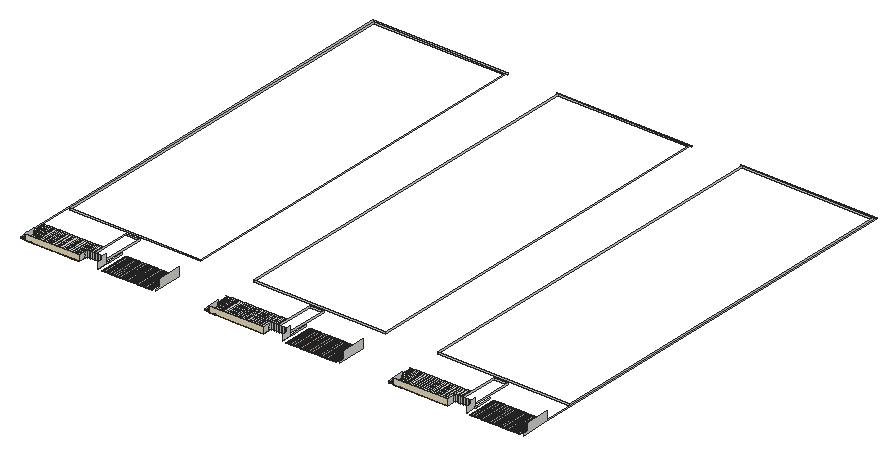
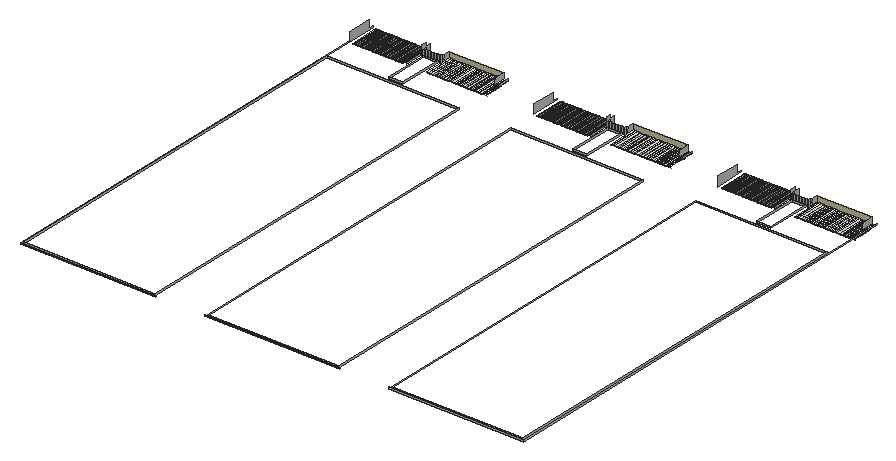
# SketchUp Ruby script. Lengths in inches.
U = 1.inch
M = Sketchup.active_model
def pt(a) = Geom::Point3d.new(a.map { |v| v * U })
def face(e, loops, mat)
  f = e.add_face(loops[0].map { |a| pt(a) })
  loops[1..].each { |l| e.add_face(l.map { |a| pt(a) }).erase! }
  f.material = f.back_material = mat if mat
  f
end
# faces: each face lists its corners as indices into pts; further lists are holes
def faces(e, pts, list, mat = nil) = list.each { |f| face(e, (f[0].is_a?(Array) ? f : [f]).map { |l| l.map { |i| pts[i] } }, mat) }
# xy, xz, yz: faces in a plane at the given z, y or x. An outline is a flat list of corners, or four numbers for a rectangle; further outlines are holes
def ring(l) = l.size == 4 ? [[l[0], l[1]], [l[2], l[1]], [l[2], l[3]], [l[0], l[3]]] : l.each_slice(2).to_a
def flat(e, list, mat, &to3) = list.each { |f| face(e, (f[0].is_a?(Array) ? f : [f]).map { |l| ring(l).map { |u, v| to3.(u, v) } }, mat) }
def xy(e, z, list, mat = nil) = flat(e, list, mat) { |x, y| [x, y, z] }
def xz(e, y, list, mat = nil) = flat(e, list, mat) { |x, z| [x, y, z] }
def yz(e, x, list, mat = nil) = flat(e, list, mat) { |y, z| [x, y, z] }
def lines(e, pts, list) = list.each { |a, b| e.add_line(pt(pts[a]), pt(pts[b])) }
# prism: a flat outline (further loops are holes) pulled along v
def prism(e, loops, v, mat = nil)
  f = face(e, loops, mat); d = Geom::Vector3d.new(v.map { |x| x * U })
  f.pushpull(f.normal.samedirection?(d) ? d.length : -d.length)
end
def box(e, o, s, mat = nil) = prism(e, [[o, [o[0] + s[0], o[1], o[2]], [o[0] + s[0], o[1] + s[1], o[2]], [o[0], o[1] + s[1], o[2]]]], [0, 0, s[2]], mat)
def at(x, y, z, deg = 0) = Geom::Transformation.translation(pt([x, y, z])) * Geom::Transformation.rotation(ORIGIN, Z_AXIS, deg.degrees)
def axes(o, x, y, z) = Geom::Transformation.new([*x, 0, *y, 0, *z, 0, *pt(o).to_a, 1])
def part(name) = M.definitions.add(name)
# library, detail: a bought-in or finely detailed component or shape, given as its bounding box
def library(name, o, s) = part(name).tap { |d| box(d.entities, o, s) }
def detail(e, o, s) = box(e.add_group.entities, o, s)
def put(e, d, t, mat = nil) = e.add_instance(d, t).tap { |i| i.material = mat if mat }
def group(e, t, mat = nil) = e.add_group.tap { |g| g.transformation = t; g.material = mat if mat }.entities
root = M.entities
M.materials.add("[Color D01]").color = [237, 225, 189]
M.materials.add("[Wood Veneer 01]").color = [51, 28, 15]
xy(root,379.5625,[[409.32,246.64,413.74,361.27],[415.32,246.64,419.74,361.27],[421.32,246.64,425.74,361.27],[427.32,246.64,431.74,361.27],[433.32,246.64,437.74,361.27],
  [439.32,246.64,443.74,361.27],[445.32,246.64,449.74,361.27],[451.32,246.64,455.74,361.27],[457.32,246.64,461.74,361.27],[463.32,246.64,467.74,361.27],
  [469.32,246.64,473.74,361.27],[475.32,246.64,479.74,361.27],[481.32,246.64,485.74,361.27],[487.32,246.64,491.74,361.27],[493.32,246.64,497.74,361.27],
  [499.32,246.64,503.74,361.27],[1142.89,246.64,1147.3,361.27],[1148.89,246.64,1153.3,361.27],[1154.89,246.64,1159.3,361.27],[1160.89,246.64,1165.3,361.27],
  [1166.89,246.64,1171.3,361.27],[1172.89,246.64,1177.3,361.27],[1178.89,246.64,1183.3,361.27],[1184.89,246.64,1189.3,361.27],[1190.89,246.64,1195.3,361.27],
  [1196.89,246.64,1201.3,361.27],[1202.89,246.64,1207.3,361.27],[1208.89,246.64,1213.3,361.27],[1214.89,246.64,1219.3,361.27],[1220.89,246.64,1225.3,361.27],
  [1226.89,246.64,1231.3,361.27],[1232.89,246.64,1237.3,361.27],[1876.45,246.64,1880.86,361.27],[1882.45,246.64,1886.86,361.27],[1888.45,246.64,1892.86,361.27],
  [1894.45,246.64,1898.86,361.27],[1900.45,246.64,1904.86,361.27],[1906.45,246.64,1910.86,361.27],[1912.45,246.64,1916.86,361.27],[1918.45,246.64,1922.86,361.27],
  [1924.45,246.64,1928.86,361.27],[1930.45,246.64,1934.86,361.27],[1936.45,246.64,1940.86,361.27],[1942.45,246.64,1946.86,361.27],[1948.45,246.64,1952.86,361.27],
  [1954.45,246.64,1958.86,361.27],[1960.45,246.64,1964.86,361.27],[1966.45,246.64,1970.86,361.27]],"[Wood Veneer 01]")
xy(root,380.0625,[[505.32,246.64,509.74,361.27],[511.32,246.64,515.74,361.27],[517.32,246.64,521.74,361.27],[523.32,246.64,527.74,361.27],[529.32,246.64,533.74,361.27],
  [535.32,246.64,539.74,361.27],[541.32,246.64,545.74,361.27],[547.32,246.64,551.74,361.27],[553.32,246.64,557.74,361.27],[559.32,246.64,563.74,361.27],
  [565.32,246.64,569.74,361.27],[1238.89,246.64,1243.3,361.27],[1244.89,246.64,1249.3,361.27],[1250.89,246.64,1255.3,361.27],[1256.89,246.64,1261.3,361.27],
  [1262.89,246.64,1267.3,361.27],[1268.89,246.64,1273.3,361.27],[1274.89,246.64,1279.3,361.27],[1280.89,246.64,1285.3,361.27],[1286.89,246.64,1291.3,361.27],
  [1292.89,246.64,1297.3,361.27],[1298.89,246.64,1303.3,361.27],[1972.45,246.64,1976.86,361.27],[1978.45,246.64,1982.86,361.27],[1984.45,246.64,1988.86,361.27],
  [1990.45,246.64,1994.86,361.27],[1996.45,246.64,2000.86,361.27],[2002.45,246.64,2006.86,361.27],[2008.45,246.64,2012.86,361.27],[2014.45,246.64,2018.86,361.27],
  [2020.45,246.64,2024.86,361.27],[2026.45,246.64,2030.86,361.27],[2032.45,246.64,2036.86,361.27]],"[Wood Veneer 01]")
xy(root,380.1875,[[571.32,246.64,575.74,361.27],[577.32,246.64,581.74,361.27],[583.32,246.64,587.74,361.27],[589.32,246.64,593.74,361.27],[595.32,246.64,599.74,361.27],
  [601.32,246.64,605.74,361.27],[1304.89,246.64,1309.3,361.27],[1310.89,246.64,1315.3,361.27],[1316.89,246.64,1321.3,361.27],[1322.89,246.64,1327.3,361.27],
  [1328.89,246.64,1333.3,361.27],[1334.89,246.64,1339.3,361.27],[2038.45,246.64,2042.86,361.27],[2044.45,246.64,2048.86,361.27],[2050.45,246.64,2054.86,361.27],
  [2056.45,246.64,2060.86,361.27],[2062.45,246.64,2066.86,361.27],[2068.45,246.64,2072.86,361.27]],"[Wood Veneer 01]")
xy(root,380.6875,[[100.08,246.64,100.18,361.27],[100.18,246.64,105.12,361.27],[105.12,246.64,108.49,361.27],[108.49,246.64,113.53,361.27],[113.53,246.64,116.9,361.27],
  [116.9,246.64,121.94,361.27],[121.94,246.64,125.32,361.27],[130.35,246.64,133.73,361.27],[133.73,246.64,138.77,361.27],[138.77,246.64,142.14,361.27],
  [142.14,246.64,147.18,361.27],[147.18,246.64,150.55,361.27],[150.55,246.64,155.59,361.27],[155.59,246.64,158.97,361.27],[158.97,246.64,164.01,361.27],
  [164.01,246.64,167.38,361.27],[167.38,246.64,172.42,361.27],[172.42,246.64,175.79,361.27],[175.79,246.64,180.83,361.27],[180.83,246.64,184.21,361.27],
  [184.21,246.64,189.24,361.27],[189.24,246.64,192.62,361.27],[192.62,246.64,197.66,361.27],[197.66,246.64,201.03,361.27],[201.03,246.64,206.07,361.27],
  [206.07,246.64,209.44,361.27],[209.44,246.64,214.48,361.27],[214.48,246.64,217.86,361.27],[217.86,246.64,222.89,361.27],[222.89,246.64,226.27,361.27],
  [226.27,246.64,231.31,361.27],[231.31,246.64,234.68,361.27],[234.68,246.64,239.72,361.27],[239.72,246.64,243.1,361.27],[243.1,246.64,248.13,361.27],
  [248.13,246.64,251.51,361.27],[251.51,246.64,256.55,361.27],[256.55,246.64,259.92,361.27],[259.92,246.64,264.96,361.27],[264.96,246.64,268.33,361.27],
  [268.33,246.64,273.37,361.27],[273.37,246.64,276.75,361.27],[276.75,246.64,281.78,361.27],[281.78,246.64,285.16,361.27],[285.16,246.64,290.2,361.27],
  [290.2,246.64,293.57,361.27],[293.57,246.64,298.61,361.27],[298.61,246.64,301.98,361.27],[301.98,246.64,307.02,361.27],[307.02,246.64,310.4,361.27],
  [310.4,246.64,315.43,361.27],[315.43,246.64,318.81,286.21],[393.95,246.64,396.57,286.21],[413.74,246.64,415.32,361.27],[419.74,246.64,421.32,361.27],
  [425.74,246.64,427.32,361.27],[431.74,246.64,433.32,361.27],[437.74,246.64,439.32,361.27],[443.74,246.64,445.32,361.27],[449.74,246.64,451.32,361.27],
  [455.74,246.64,457.32,361.27],[461.74,246.64,463.32,361.27],[467.74,246.64,469.32,361.27],[473.74,246.64,475.32,361.27],[479.74,246.64,481.32,361.27],
  [485.74,246.64,487.32,361.27],[491.74,246.64,493.32,361.27],[497.74,246.64,499.32,361.27],[503.74,246.64,505.32,361.27],[509.74,246.64,511.32,361.27],
  [515.74,246.64,517.32,361.27],[521.74,246.64,523.32,361.27],[527.74,246.64,529.32,361.27],[533.74,246.64,535.32,361.27],[539.74,246.64,541.32,361.27],
  [545.74,246.64,547.32,361.27],[551.74,246.64,553.32,361.27],[557.74,246.64,559.32,361.27],[563.74,246.64,565.32,361.27],[569.74,246.64,571.32,361.27],
  [575.74,246.64,577.32,361.27],[581.74,246.64,583.32,361.27],[587.74,246.64,589.32,361.27],[593.74,246.64,595.32,361.27],[599.74,246.64,601.32,361.27],
  [605.74,246.64,609.07,361.27],[833.64,246.64,833.74,361.27],[833.74,246.64,838.68,361.27],[838.68,246.64,842.05,361.27],[842.05,246.64,847.09,361.27],
  [847.09,246.64,850.47,361.27],[850.47,246.64,855.5,361.27],[855.5,246.64,858.88,361.27],[863.92,246.64,867.29,361.27],[867.29,246.64,872.33,361.27],
  [872.33,246.64,875.7,361.27],[875.7,246.64,880.74,361.27],[880.74,246.64,884.12,361.27],[884.12,246.64,889.16,361.27],[889.16,246.64,892.53,361.27],
  [892.53,246.64,897.57,361.27],[897.57,246.64,900.94,361.27],[900.94,246.64,905.98,361.27],[905.98,246.64,909.36,361.27],[909.36,246.64,914.39,361.27],
  [914.39,246.64,917.77,361.27],[917.77,246.64,922.81,361.27],[922.81,246.64,926.18,361.27],[926.18,246.64,931.22,361.27],[931.22,246.64,934.59,361.27],
  [934.59,246.64,939.63,361.27],[939.63,246.64,943.01,361.27],[943.01,246.64,948.04,361.27],[948.04,246.64,951.42,361.27],[951.42,246.64,956.46,361.27],
  [956.46,246.64,959.83,361.27],[959.83,246.64,964.87,361.27],[964.87,246.64,968.24,361.27],[968.24,246.64,973.28,361.27],[973.28,246.64,976.66,361.27],
  [976.66,246.64,981.7,361.27],[981.7,246.64,985.07,361.27],[985.07,246.64,990.11,361.27],[990.11,246.64,993.48,361.27],[993.48,246.64,998.52,361.27],
  [998.52,246.64,1001.9,361.27],[1001.9,246.64,1006.93,361.27],[1006.93,246.64,1010.31,361.27],[1010.31,246.64,1015.35,361.27],[1015.35,246.64,1018.72,361.27],
  [1018.72,246.64,1023.76,361.27],[1023.76,246.64,1027.13,361.27],[1027.13,246.64,1032.17,361.27],[1032.17,246.64,1035.55,361.27],[1035.55,246.64,1040.58,361.27],
  [1040.58,246.64,1043.96,361.27],[1043.96,246.64,1049,361.27],[1049,246.64,1052.37,286.21],[1127.51,246.64,1130.14,286.21],[1147.3,246.64,1148.89,361.27],
  [1153.3,246.64,1154.89,361.27],[1159.3,246.64,1160.89,361.27],[1165.3,246.64,1166.89,361.27],[1171.3,246.64,1172.89,361.27],[1177.3,246.64,1178.89,361.27],
  [1183.3,246.64,1184.89,361.27],[1189.3,246.64,1190.89,361.27],[1195.3,246.64,1196.89,361.27],[1201.3,246.64,1202.89,361.27],[1207.3,246.64,1208.89,361.27],
  [1213.3,246.64,1214.89,361.27],[1219.3,246.64,1220.89,361.27],[1225.3,246.64,1226.89,361.27],[1231.3,246.64,1232.89,361.27],[1237.3,246.64,1238.89,361.27],
  [1243.3,246.64,1244.89,361.27],[1249.3,246.64,1250.89,361.27],[1255.3,246.64,1256.89,361.27],[1261.3,246.64,1262.89,361.27],[1267.3,246.64,1268.89,361.27],
  [1273.3,246.64,1274.89,361.27],[1279.3,246.64,1280.89,361.27],[1285.3,246.64,1286.89,361.27],[1291.3,246.64,1292.89,361.27],[1297.3,246.64,1298.89,361.27],
  [1303.3,246.64,1304.89,361.27],[1309.3,246.64,1310.89,361.27],[1315.3,246.64,1316.89,361.27],[1321.3,246.64,1322.89,361.27],[1327.3,246.64,1328.89,361.27],
  [1333.3,246.64,1334.89,361.27],[1339.3,246.64,1342.64,361.27],[1567.2,246.64,1567.3,361.27],[1567.3,246.64,1572.24,361.27],[1572.24,246.64,1575.62,361.27],
  [1575.62,246.64,1580.65,361.27],[1580.65,246.64,1584.03,361.27],[1584.03,246.64,1589.07,361.27],[1589.07,246.64,1592.44,361.27],[1597.48,246.64,1600.85,361.27],
  [1600.85,246.64,1605.89,361.27],[1605.89,246.64,1609.27,361.27],[1609.27,246.64,1614.3,361.27],[1614.3,246.64,1617.68,361.27],[1617.68,246.64,1622.72,361.27],
  [1622.72,246.64,1626.09,361.27],[1626.09,246.64,1631.13,361.27],[1631.13,246.64,1634.51,361.27],[1634.51,246.64,1639.54,361.27],[1639.54,246.64,1642.92,361.27],
  [1642.92,246.64,1647.96,361.27],[1647.96,246.64,1651.33,361.27],[1651.33,246.64,1656.37,361.27],[1656.37,246.64,1659.74,361.27],[1659.74,246.64,1664.78,361.27],
  [1664.78,246.64,1668.16,361.27],[1668.16,246.64,1673.19,361.27],[1673.19,246.64,1676.57,361.27],[1676.57,246.64,1681.61,361.27],[1681.61,246.64,1684.98,361.27],
  [1684.98,246.64,1690.02,361.27],[1690.02,246.64,1693.39,361.27],[1693.39,246.64,1698.43,361.27],[1698.43,246.64,1701.81,361.27],[1701.81,246.64,1706.85,361.27],
  [1706.85,246.64,1710.22,361.27],[1710.22,246.64,1715.26,361.27],[1715.26,246.64,1718.63,361.27],[1718.63,246.64,1723.67,361.27],[1723.67,246.64,1727.05,361.27],
  [1727.05,246.64,1732.08,361.27],[1732.08,246.64,1735.46,361.27],[1735.46,246.64,1740.5,361.27],[1740.5,246.64,1743.87,361.27],[1743.87,246.64,1748.91,361.27],
  [1748.91,246.64,1752.28,361.27],[1752.28,246.64,1757.32,361.27],[1757.32,246.64,1760.7,361.27],[1760.7,246.64,1765.73,361.27],[1765.73,246.64,1769.11,361.27],
  [1769.11,246.64,1774.15,361.27],[1774.15,246.64,1777.52,361.27],[1777.52,246.64,1782.56,361.27],[1782.56,246.64,1785.93,286.21],[1861.07,246.64,1863.7,286.21],
  [1880.86,246.64,1882.45,361.27],[1886.86,246.64,1888.45,361.27],[1892.86,246.64,1894.45,361.27],[1898.86,246.64,1900.45,361.27],[1904.86,246.64,1906.45,361.27],
  [1910.86,246.64,1912.45,361.27],[1916.86,246.64,1918.45,361.27],[1922.86,246.64,1924.45,361.27],[1928.86,246.64,1930.45,361.27],[1934.86,246.64,1936.45,361.27],
  [1940.86,246.64,1942.45,361.27],[1946.86,246.64,1948.45,361.27],[1952.86,246.64,1954.45,361.27],[1958.86,246.64,1960.45,361.27],[1964.86,246.64,1966.45,361.27],
  [1970.86,246.64,1972.45,361.27],[1976.86,246.64,1978.45,361.27],[1982.86,246.64,1984.45,361.27],[1988.86,246.64,1990.45,361.27],[1994.86,246.64,1996.45,361.27],
  [2000.86,246.64,2002.45,361.27],[2006.86,246.64,2008.45,361.27],[2012.86,246.64,2014.45,361.27],[2018.86,246.64,2020.45,361.27],[2024.86,246.64,2026.45,361.27],
  [2030.86,246.64,2032.45,361.27],[2036.86,246.64,2038.45,361.27],[2042.86,246.64,2044.45,361.27],[2048.86,246.64,2050.45,361.27],[2054.86,246.64,2056.45,361.27],
  [2060.86,246.64,2062.45,361.27],[2066.86,246.64,2068.45,361.27],[2072.86,246.64,2076.2,361.27]])
xy(root,380.9375,[[125.32,246.64,130.35,361.27],[858.88,246.64,863.92,361.27],[1592.44,246.64,1597.48,361.27]])
xz(root,246.64,[[100.18,380.6875,125.32,380.6875,125.32,380.9375,130.35,380.9375,130.35,380.6875,318.81,380.6875,318.81,403.1875,100.18,403.1875],[833.74,380.6875,858.88,380.6875,858.88,380.9375,863.92,380.9375,863.92,380.6875,1052.37,380.6875,1052.37,403.1875,833.74,403.1875],[1567.3,380.6875,1592.44,380.6875,1592.44,380.9375,1597.48,380.9375,1597.48,380.6875,1785.93,380.6875,1785.93,403.1875,1567.3,403.1875]],"[Color D01]")
xz(root,286.21,[[315.43,380.6875,318.81,380.6875,318.81,403.1875,315.68,403.1875,315.68,409.375,315.43,409.375],[393.95,380.6875,396.57,386.6875],[1049,380.6875,1052.37,380.6875,1052.37,403.1875,1049.24,403.1875,1049.24,409.375,1049,409.375],[1127.51,380.6875,1130.14,386.6875],[1782.56,380.6875,1785.93,380.6875,1785.93,403.1875,1782.8,403.1875,1782.8,409.375,1782.56,409.375],
  [1861.07,380.6875,1863.7,386.6875]])
xz(root,293.45,[[328.03,380.6875,382.74,386.6875],[1061.59,380.6875,1116.3,386.6875],[1795.15,380.6875,1849.87,386.6875]])
xz(root,465.02,[[328.03,380.6875,382.74,386.6875],[1061.59,380.6875,1116.3,386.6875],[1795.15,380.6875,1849.87,386.6875]])
xz(root,483.79,[[90.36,380.6875,614.76,386.6875],[823.93,380.6875,1348.32,386.6875],[1557.49,380.6875,2081.89,386.6875]])
xz(root,1996.66,[[90.36,380.6875,614.76,386.6875],[823.93,380.6875,1348.32,386.6875],[1557.49,380.6875,2081.89,386.6875]])
xz(root,2003.89,[[83.125,380.6875,622,386.6875],[816.6875,380.6875,1355.5625,386.6875],[1550.25,380.6875,2089.125,386.6875]])
yz(root,83.125,[[246.64,380.6875,293.46,386.6875],[293.46,380.6875,2003.89,386.6875]])
yz(root,90.36,[[483.79,380.6875,1996.66,386.6875]])
yz(root,100.18,[[246.64,380.6875,293.45,380.6875,293.45,402.5,255.92,402.5,255.92,403.1875,246.64,403.1875],[293.45,380.6875,293.46,402.5]])
yz(root,125.32,[[246.64,380.6875,361.27,380.9375]])
yz(root,130.35,[[246.64,380.6875,286.21,380.9375],[286.21,380.6875,293.45,380.9375],[293.45,380.6875,361.27,380.9375]])
yz(root,315.43,[[286.21,380.6875,293.45,409.375]])
yz(root,318.81,[[246.64,380.6875,271.96,403.1875],[271.96,380.6875,286.21,403.1875]])
yz(root,324.81,[[282.52,380.6875,286.21,403.1875]])
yz(root,328.03,[[293.45,380.6875,465.02,386.6875]])
yz(root,330.81,[[282.52,380.6875,286.21,403.1875]])
yz(root,336.81,[[282.52,380.6875,286.21,403.1875]])
yz(root,342.81,[[282.52,380.6875,286.21,403.1875]])
yz(root,348.81,[[283.46,380.6875,286.21,403.1875]])
yz(root,354.81,[[283.46,380.6875,286.21,403.1875]])
yz(root,360.81,[[283.46,380.6875,286.21,403.1875]])
yz(root,366.81,[[283.46,380.6875,286.21,403.1875]])
yz(root,372.81,[[283.46,380.6875,286.21,403.1875]])
yz(root,378.81,[[283.46,380.6875,286.21,403.1875]])
yz(root,382.74,[[293.45,380.6875,465.02,386.6875]])
yz(root,384.81,[[283.46,380.6875,286.21,403.1875]])
yz(root,390.12,[[272.89,380.6875,286.21,403.1875]])
yz(root,393.95,[[246.64,380.6875,246.64,403.1875,266.49,403.1875,266.49,416.75,286.21,416.75,286.21,380.6875]])
yz(root,396.57,[[286.21,380.6875,293.45,386.6875],[293.45,380.6875,361.27,386.6875]])
yz(root,413.74,[[246.64,379.5625,361.27,380.6875]])
yz(root,415.32,[[246.64,379.5625,361.27,380.6875]])
yz(root,419.74,[[246.64,379.5625,361.27,380.6875]])
yz(root,421.32,[[246.64,379.5625,361.27,380.6875]])
yz(root,425.74,[[246.64,379.5625,361.27,380.6875]])
yz(root,427.32,[[246.64,379.5625,361.27,380.6875]])
yz(root,431.74,[[246.64,379.5625,361.27,380.6875]])
yz(root,433.32,[[246.64,379.5625,361.27,380.6875]])
yz(root,437.74,[[246.64,379.5625,361.27,380.6875]])
yz(root,439.32,[[246.64,379.5625,361.27,380.6875]])
yz(root,443.74,[[246.64,379.5625,361.27,380.6875]])
yz(root,445.32,[[246.64,379.5625,361.27,380.6875]])
yz(root,449.74,[[246.64,379.5625,361.27,380.6875]])
yz(root,451.32,[[246.64,379.5625,361.27,380.6875]])
yz(root,455.74,[[246.64,379.5625,361.27,380.6875]])
yz(root,457.32,[[246.64,379.5625,361.27,380.6875]])
yz(root,461.74,[[246.64,379.5625,361.27,380.6875]])
yz(root,463.32,[[246.64,379.5625,361.27,380.6875]])
yz(root,467.74,[[246.64,379.5625,361.27,380.6875]])
yz(root,469.32,[[246.64,379.5625,361.27,380.6875]])
yz(root,473.74,[[246.64,379.5625,361.27,380.6875]])
yz(root,475.32,[[246.64,379.5625,361.27,380.6875]])
yz(root,479.74,[[246.64,379.5625,361.27,380.6875]])
yz(root,481.32,[[246.64,379.5625,361.27,380.6875]])
yz(root,485.74,[[246.64,379.5625,361.27,380.6875]])
yz(root,487.32,[[246.64,379.5625,361.27,380.6875]])
yz(root,491.74,[[246.64,379.5625,361.27,380.6875]])
yz(root,493.32,[[246.64,379.5625,361.27,380.6875]])
yz(root,497.74,[[246.64,379.5625,361.27,380.6875]])
yz(root,499.32,[[246.64,379.5625,361.27,380.6875]])
yz(root,503.74,[[246.64,379.5625,361.27,380.6875]])
yz(root,505.32,[[246.64,380.0625,361.27,380.6875]])
yz(root,509.74,[[246.64,380.0625,361.27,380.6875]])
yz(root,511.32,[[246.64,380.0625,361.27,380.6875]])
yz(root,515.74,[[246.64,380.0625,361.27,380.6875]])
yz(root,517.32,[[246.64,380.0625,361.27,380.6875]])
yz(root,521.74,[[246.64,380.0625,361.27,380.6875]])
yz(root,523.32,[[246.64,380.0625,361.27,380.6875]])
yz(root,527.74,[[246.64,380.0625,361.27,380.6875]])
yz(root,529.32,[[246.64,380.0625,361.27,380.6875]])
yz(root,533.74,[[246.64,380.0625,361.27,380.6875]])
yz(root,535.32,[[246.64,380.0625,361.27,380.6875]])
yz(root,539.74,[[246.64,380.0625,361.27,380.6875]])
yz(root,541.32,[[246.64,380.0625,361.27,380.6875]])
yz(root,545.74,[[246.64,380.0625,361.27,380.6875]])
yz(root,547.32,[[246.64,380.0625,361.27,380.6875]])
yz(root,551.74,[[246.64,380.0625,361.27,380.6875]])
yz(root,553.32,[[246.64,380.0625,361.27,380.6875]])
yz(root,557.74,[[246.64,380.0625,361.27,380.6875]])
yz(root,559.32,[[246.64,380.0625,361.27,380.6875]])
yz(root,563.74,[[246.64,380.0625,361.27,380.6875]])
yz(root,565.32,[[246.64,380.0625,361.27,380.6875]])
yz(root,569.74,[[246.64,380.0625,361.27,380.6875]])
yz(root,571.32,[[246.64,380.1875,361.27,380.6875]])
yz(root,575.74,[[246.64,380.1875,361.27,380.6875]])
yz(root,577.32,[[246.64,380.1875,361.27,380.6875]])
yz(root,581.74,[[246.64,380.1875,361.27,380.6875]])
yz(root,583.32,[[246.64,380.1875,361.27,380.6875]])
yz(root,587.74,[[246.64,380.1875,361.27,380.6875]])
yz(root,589.32,[[246.64,380.1875,361.27,380.6875]])
yz(root,593.74,[[246.64,380.1875,361.27,380.6875]])
yz(root,595.32,[[246.64,380.1875,361.27,380.6875]])
yz(root,599.74,[[246.64,380.1875,361.27,380.6875]])
yz(root,601.32,[[246.64,380.1875,361.27,380.6875]])
yz(root,605.74,[[246.64,380.1875,361.27,380.6875]])
yz(root,614.76,[[483.79,380.6875,1996.66,386.6875]])
yz(root,622,[[246.64,380.6875,361.27,380.6875,361.27,416.75,266.43,416.75,266.43,386.6875,246.64,386.6875]])
yz(root,816.6875,[[246.64,380.6875,293.46,386.6875]])
yz(root,823.93,[[483.79,380.6875,1996.66,386.6875]])
yz(root,833.74,[[246.64,380.6875,293.45,380.6875,293.45,402.5,255.92,402.5,255.92,403.1875,246.64,403.1875],[293.45,380.6875,293.46,402.5]])
yz(root,858.88,[[246.64,380.6875,361.27,380.9375]])
yz(root,863.92,[[246.64,380.6875,286.21,380.9375],[286.21,380.6875,293.45,380.9375],[293.45,380.6875,361.27,380.9375]])
yz(root,1049,[[286.21,380.6875,293.45,409.375]])
yz(root,1052.37,[[246.64,380.6875,271.96,403.1875],[271.96,380.6875,286.21,403.1875]])
yz(root,1058.37,[[282.52,380.6875,286.21,403.1875]])
yz(root,1061.59,[[293.45,380.6875,465.02,386.6875]])
yz(root,1064.37,[[282.52,380.6875,286.21,403.1875]])
yz(root,1070.37,[[282.52,380.6875,286.21,403.1875]])
yz(root,1076.37,[[282.52,380.6875,286.21,403.1875]])
yz(root,1082.37,[[283.46,380.6875,286.21,403.1875]])
yz(root,1088.37,[[283.46,380.6875,286.21,403.1875]])
yz(root,1094.37,[[283.46,380.6875,286.21,403.1875]])
yz(root,1100.37,[[283.46,380.6875,286.21,403.1875]])
yz(root,1106.37,[[283.46,380.6875,286.21,403.1875]])
yz(root,1112.37,[[283.46,380.6875,286.21,403.1875]])
yz(root,1116.3,[[293.45,380.6875,465.02,386.6875]])
yz(root,1118.37,[[283.46,380.6875,286.21,403.1875]])
yz(root,1123.68,[[272.89,380.6875,286.21,403.1875]])
yz(root,1127.51,[[246.64,380.6875,246.64,403.1875,266.49,403.1875,266.49,416.75,286.21,416.75,286.21,380.6875]])
yz(root,1130.14,[[286.21,380.6875,293.45,386.6875],[293.45,380.6875,361.27,386.6875]])
yz(root,1147.3,[[246.64,379.5625,361.27,380.6875]])
yz(root,1148.89,[[246.64,379.5625,361.27,380.6875]])
yz(root,1153.3,[[246.64,379.5625,361.27,380.6875]])
yz(root,1154.89,[[246.64,379.5625,361.27,380.6875]])
yz(root,1159.3,[[246.64,379.5625,361.27,380.6875]])
yz(root,1160.89,[[246.64,379.5625,361.27,380.6875]])
yz(root,1165.3,[[246.64,379.5625,361.27,380.6875]])
yz(root,1166.89,[[246.64,379.5625,361.27,380.6875]])
yz(root,1171.3,[[246.64,379.5625,361.27,380.6875]])
yz(root,1172.89,[[246.64,379.5625,361.27,380.6875]])
yz(root,1177.3,[[246.64,379.5625,361.27,380.6875]])
yz(root,1178.89,[[246.64,379.5625,361.27,380.6875]])
yz(root,1183.3,[[246.64,379.5625,361.27,380.6875]])
yz(root,1184.89,[[246.64,379.5625,361.27,380.6875]])
yz(root,1189.3,[[246.64,379.5625,361.27,380.6875]])
yz(root,1190.89,[[246.64,379.5625,361.27,380.6875]])
yz(root,1195.3,[[246.64,379.5625,361.27,380.6875]])
yz(root,1196.89,[[246.64,379.5625,361.27,380.6875]])
yz(root,1201.3,[[246.64,379.5625,361.27,380.6875]])
yz(root,1202.89,[[246.64,379.5625,361.27,380.6875]])
yz(root,1207.3,[[246.64,379.5625,361.27,380.6875]])
yz(root,1208.89,[[246.64,379.5625,361.27,380.6875]])
yz(root,1213.3,[[246.64,379.5625,361.27,380.6875]])
yz(root,1214.89,[[246.64,379.5625,361.27,380.6875]])
yz(root,1219.3,[[246.64,379.5625,361.27,380.6875]])
yz(root,1220.89,[[246.64,379.5625,361.27,380.6875]])
yz(root,1225.3,[[246.64,379.5625,361.27,380.6875]])
yz(root,1226.89,[[246.64,379.5625,361.27,380.6875]])
yz(root,1231.3,[[246.64,379.5625,361.27,380.6875]])
yz(root,1232.89,[[246.64,379.5625,361.27,380.6875]])
yz(root,1237.3,[[246.64,379.5625,361.27,380.6875]])
yz(root,1238.89,[[246.64,380.0625,361.27,380.6875]])
yz(root,1243.3,[[246.64,380.0625,361.27,380.6875]])
yz(root,1244.89,[[246.64,380.0625,361.27,380.6875]])
yz(root,1249.3,[[246.64,380.0625,361.27,380.6875]])
yz(root,1250.89,[[246.64,380.0625,361.27,380.6875]])
yz(root,1255.3,[[246.64,380.0625,361.27,380.6875]])
yz(root,1256.89,[[246.64,380.0625,361.27,380.6875]])
yz(root,1261.3,[[246.64,380.0625,361.27,380.6875]])
yz(root,1262.89,[[246.64,380.0625,361.27,380.6875]])
yz(root,1267.3,[[246.64,380.0625,361.27,380.6875]])
yz(root,1268.89,[[246.64,380.0625,361.27,380.6875]])
yz(root,1273.3,[[246.64,380.0625,361.27,380.6875]])
yz(root,1274.89,[[246.64,380.0625,361.27,380.6875]])
yz(root,1279.3,[[246.64,380.0625,361.27,380.6875]])
yz(root,1280.89,[[246.64,380.0625,361.27,380.6875]])
yz(root,1285.3,[[246.64,380.0625,361.27,380.6875]])
yz(root,1286.89,[[246.64,380.0625,361.27,380.6875]])
yz(root,1291.3,[[246.64,380.0625,361.27,380.6875]])
yz(root,1292.89,[[246.64,380.0625,361.27,380.6875]])
yz(root,1297.3,[[246.64,380.0625,361.27,380.6875]])
yz(root,1298.89,[[246.64,380.0625,361.27,380.6875]])
yz(root,1303.3,[[246.64,380.0625,361.27,380.6875]])
yz(root,1304.89,[[246.64,380.1875,361.27,380.6875]])
yz(root,1309.3,[[246.64,380.1875,361.27,380.6875]])
yz(root,1310.89,[[246.64,380.1875,361.27,380.6875]])
yz(root,1315.3,[[246.64,380.1875,361.27,380.6875]])
yz(root,1316.89,[[246.64,380.1875,361.27,380.6875]])
yz(root,1321.3,[[246.64,380.1875,361.27,380.6875]])
yz(root,1322.89,[[246.64,380.1875,361.27,380.6875]])
yz(root,1327.3,[[246.64,380.1875,361.27,380.6875]])
yz(root,1328.89,[[246.64,380.1875,361.27,380.6875]])
yz(root,1333.3,[[246.64,380.1875,361.27,380.6875]])
yz(root,1334.89,[[246.64,380.1875,361.27,380.6875]])
yz(root,1339.3,[[246.64,380.1875,361.27,380.6875]])
yz(root,1348.32,[[483.79,380.6875,1996.66,386.6875]])
yz(root,1355.5625,[[246.64,380.6875,361.27,380.6875,361.27,416.75,266.43,416.75,266.43,386.6875,246.64,386.6875]])
yz(root,1550.25,[[246.64,380.6875,293.46,386.6875]])
yz(root,1557.49,[[483.79,380.6875,1996.66,386.6875]])
yz(root,1567.3,[[246.64,380.6875,293.45,380.6875,293.45,402.5,255.92,402.5,255.92,403.1875,246.64,403.1875],[293.45,380.6875,293.46,402.5]])
yz(root,1592.44,[[246.64,380.6875,361.27,380.9375]])
yz(root,1597.48,[[246.64,380.6875,286.21,380.9375],[286.21,380.6875,293.45,380.9375],[293.45,380.6875,361.27,380.9375]])
yz(root,1782.56,[[286.21,380.6875,293.45,409.375]])
yz(root,1785.93,[[246.64,380.6875,271.96,403.1875],[271.96,380.6875,286.21,403.1875]])
yz(root,1791.93,[[282.52,380.6875,286.21,403.1875]])
yz(root,1795.15,[[293.45,380.6875,465.02,386.6875]])
yz(root,1797.93,[[282.52,380.6875,286.21,403.1875]])
yz(root,1803.93,[[282.52,380.6875,286.21,403.1875]])
yz(root,1809.93,[[282.52,380.6875,286.21,403.1875]])
yz(root,1815.93,[[283.46,380.6875,286.21,403.1875]])
yz(root,1821.93,[[283.46,380.6875,286.21,403.1875]])
yz(root,1827.93,[[283.46,380.6875,286.21,403.1875]])
yz(root,1833.93,[[283.46,380.6875,286.21,403.1875]])
yz(root,1839.93,[[283.46,380.6875,286.21,403.1875]])
yz(root,1845.93,[[283.46,380.6875,286.21,403.1875]])
yz(root,1849.87,[[293.45,380.6875,465.02,386.6875]])
yz(root,1851.93,[[283.46,380.6875,286.21,403.1875]])
yz(root,1857.25,[[272.89,380.6875,286.21,403.1875]])
yz(root,1861.07,[[246.64,380.6875,246.64,403.1875,266.49,403.1875,266.49,416.75,286.21,416.75,286.21,380.6875]])
yz(root,1863.7,[[286.21,380.6875,293.45,386.6875],[293.45,380.6875,361.27,386.6875]])
yz(root,1880.86,[[246.64,379.5625,361.27,380.6875]])
yz(root,1882.45,[[246.64,379.5625,361.27,380.6875]])
yz(root,1886.86,[[246.64,379.5625,361.27,380.6875]])
yz(root,1888.45,[[246.64,379.5625,361.27,380.6875]])
yz(root,1892.86,[[246.64,379.5625,361.27,380.6875]])
yz(root,1894.45,[[246.64,379.5625,361.27,380.6875]])
yz(root,1898.86,[[246.64,379.5625,361.27,380.6875]])
yz(root,1900.45,[[246.64,379.5625,361.27,380.6875]])
yz(root,1904.86,[[246.64,379.5625,361.27,380.6875]])
yz(root,1906.45,[[246.64,379.5625,361.27,380.6875]])
yz(root,1910.86,[[246.64,379.5625,361.27,380.6875]])
yz(root,1912.45,[[246.64,379.5625,361.27,380.6875]])
yz(root,1916.86,[[246.64,379.5625,361.27,380.6875]])
yz(root,1918.45,[[246.64,379.5625,361.27,380.6875]])
yz(root,1922.86,[[246.64,379.5625,361.27,380.6875]])
yz(root,1924.45,[[246.64,379.5625,361.27,380.6875]])
yz(root,1928.86,[[246.64,379.5625,361.27,380.6875]])
yz(root,1930.45,[[246.64,379.5625,361.27,380.6875]])
yz(root,1934.86,[[246.64,379.5625,361.27,380.6875]])
yz(root,1936.45,[[246.64,379.5625,361.27,380.6875]])
yz(root,1940.86,[[246.64,379.5625,361.27,380.6875]])
yz(root,1942.45,[[246.64,379.5625,361.27,380.6875]])
yz(root,1946.86,[[246.64,379.5625,361.27,380.6875]])
yz(root,1948.45,[[246.64,379.5625,361.27,380.6875]])
yz(root,1952.86,[[246.64,379.5625,361.27,380.6875]])
yz(root,1954.45,[[246.64,379.5625,361.27,380.6875]])
yz(root,1958.86,[[246.64,379.5625,361.27,380.6875]])
yz(root,1960.45,[[246.64,379.5625,361.27,380.6875]])
yz(root,1964.86,[[246.64,379.5625,361.27,380.6875]])
yz(root,1966.45,[[246.64,379.5625,361.27,380.6875]])
yz(root,1970.86,[[246.64,379.5625,361.27,380.6875]])
yz(root,1972.45,[[246.64,380.0625,361.27,380.6875]])
yz(root,1976.86,[[246.64,380.0625,361.27,380.6875]])
yz(root,1978.45,[[246.64,380.0625,361.27,380.6875]])
yz(root,1982.86,[[246.64,380.0625,361.27,380.6875]])
yz(root,1984.45,[[246.64,380.0625,361.27,380.6875]])
yz(root,1988.86,[[246.64,380.0625,361.27,380.6875]])
yz(root,1990.45,[[246.64,380.0625,361.27,380.6875]])
yz(root,1994.86,[[246.64,380.0625,361.27,380.6875]])
yz(root,1996.45,[[246.64,380.0625,361.27,380.6875]])
yz(root,2000.86,[[246.64,380.0625,361.27,380.6875]])
yz(root,2002.45,[[246.64,380.0625,361.27,380.6875]])
yz(root,2006.86,[[246.64,380.0625,361.27,380.6875]])
yz(root,2008.45,[[246.64,380.0625,361.27,380.6875]])
yz(root,2012.86,[[246.64,380.0625,361.27,380.6875]])
yz(root,2014.45,[[246.64,380.0625,361.27,380.6875]])
yz(root,2018.86,[[246.64,380.0625,361.27,380.6875]])
yz(root,2020.45,[[246.64,380.0625,361.27,380.6875]])
yz(root,2024.86,[[246.64,380.0625,361.27,380.6875]])
yz(root,2026.45,[[246.64,380.0625,361.27,380.6875]])
yz(root,2030.86,[[246.64,380.0625,361.27,380.6875]])
yz(root,2032.45,[[246.64,380.0625,361.27,380.6875]])
yz(root,2036.86,[[246.64,380.0625,361.27,380.6875]])
yz(root,2038.45,[[246.64,380.1875,361.27,380.6875]])
yz(root,2042.86,[[246.64,380.1875,361.27,380.6875]])
yz(root,2044.45,[[246.64,380.1875,361.27,380.6875]])
yz(root,2048.86,[[246.64,380.1875,361.27,380.6875]])
yz(root,2050.45,[[246.64,380.1875,361.27,380.6875]])
yz(root,2054.86,[[246.64,380.1875,361.27,380.6875]])
yz(root,2056.45,[[246.64,380.1875,361.27,380.6875]])
yz(root,2060.86,[[246.64,380.1875,361.27,380.6875]])
yz(root,2062.45,[[246.64,380.1875,361.27,380.6875]])
yz(root,2066.86,[[246.64,380.1875,361.27,380.6875]])
yz(root,2068.45,[[246.64,380.1875,361.27,380.6875]])
yz(root,2072.86,[[246.64,380.1875,361.27,380.6875]])
yz(root,2081.89,[[483.79,380.6875,1996.66,386.6875]])
yz(root,2089.125,[[246.64,380.6875,361.27,380.6875,361.27,416.75,266.43,416.75,266.43,386.6875,246.64,386.6875],[361.27,380.6875,2003.89,386.6875]])
p = [[830.27,286.21,380.6875],[830.27,293.45,380.6875],[830.27,246.64,380.6875],[825.23,361.27,380.6875],[825.23,246.64,380.6875],[830.27,361.27,380.6875],
  [821.85,286.21,380.6875],[821.85,293.45,380.6875],[821.85,246.64,380.6875],[816.82,361.27,380.6875],[816.82,246.64,380.6875],[821.85,361.27,380.6875],
  [813.44,286.21,380.6875],[813.44,293.45,380.6875],[808.4,361.27,380.6875],[813.44,361.27,380.6875],[1563.83,286.21,380.6875],[1563.83,293.45,380.6875],
  [1563.83,246.64,380.6875],[1558.79,361.27,380.6875],[1558.79,246.64,380.6875],[1563.83,361.27,380.6875],[1555.42,286.21,380.6875],[1555.42,293.45,380.6875],
  [1555.42,246.64,380.6875],[1541.97,361.27,380.6875],[1547,361.27,380.6875],[1547,293.45,380.6875],[1547,286.21,380.6875],[1555.42,361.27,380.6875],
  [1550.38,361.27,380.6875],[1550.38,246.64,380.6875],[91.67,361.27,380.6875],[91.67,246.64,380.6875],[96.7,293.45,380.6875],[96.7,361.27,380.6875],
  [88.29,246.64,380.6875],[88.29,286.21,380.6875],[96.7,246.64,380.6875],[96.7,286.21,380.6875],[88.29,293.45,380.6875],[79.88,293.45,380.6875],
  [79.88,361.27,380.6875],[79.88,286.21,380.6875],[74.84,361.27,380.6875],[88.29,361.27,380.6875],[83.25,361.27,380.6875],[83.25,246.64,380.6875]]
lines(root,p,[[0,1],[2,0],[3,4],[3,5],[1,5],[6,7],[8,6],[9,10],[9,11],[7,11],[12,13],[14,15],
  [16,17],[18,16],[19,20],[17,21],[22,23],[24,22],[19,21],[25,26],[27,26],[28,27],[23,29],[30,31],
  [30,29],[32,33],[34,35],[32,35],[36,37],[38,39],[37,40],[39,34],[41,42],[43,41],[44,42],[40,45],
  [46,47],[46,45]])
